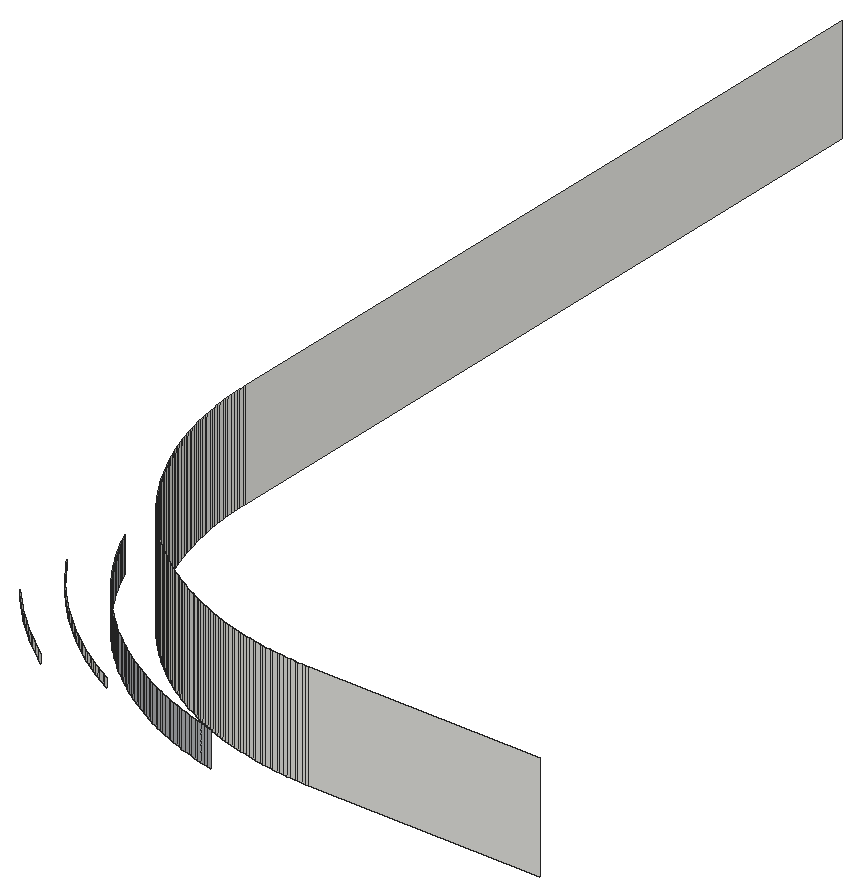
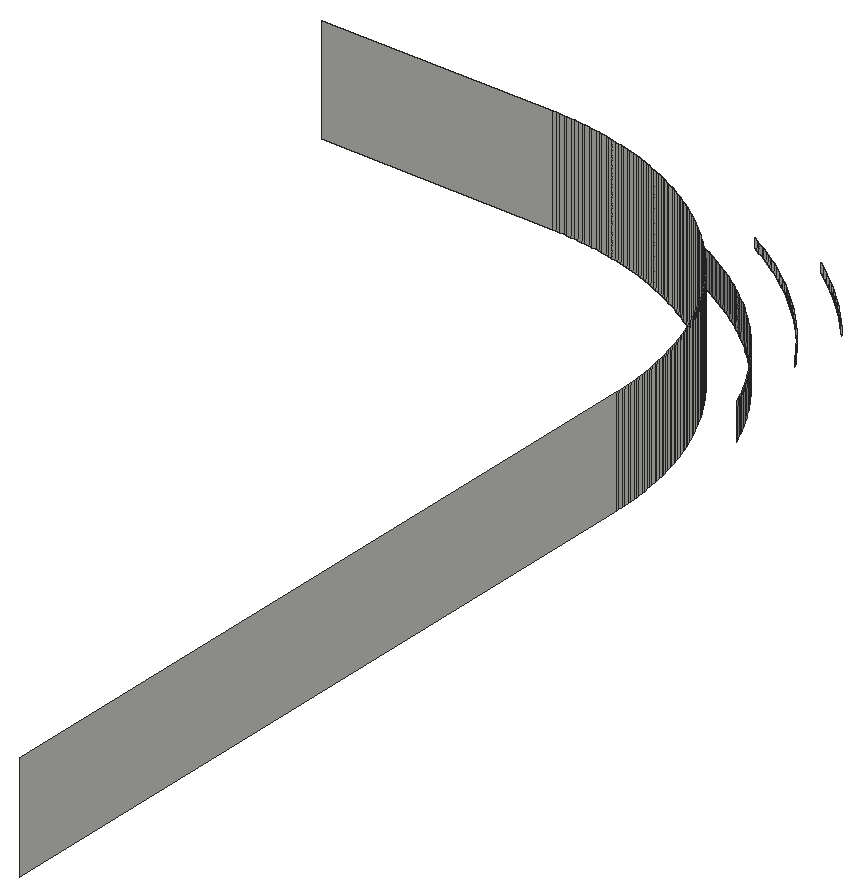
# SketchUp Ruby script. Lengths in inches.
U = 1.inch
M = Sketchup.active_model
def pt(a) = Geom::Point3d.new(a.map { |v| v * U })
def face(e, loops, mat)
  f = e.add_face(loops[0].map { |a| pt(a) })
  loops[1..].each { |l| e.add_face(l.map { |a| pt(a) }).erase! }
  f.material = f.back_material = mat if mat
  f
end
# faces: each face lists its corners as indices into pts; further lists are holes
def faces(e, pts, list, mat = nil) = list.each { |f| face(e, (f[0].is_a?(Array) ? f : [f]).map { |l| l.map { |i| pts[i] } }, mat) }
# xy, xz, yz: faces in a plane at the given z, y or x. An outline is a flat list of corners, or four numbers for a rectangle; further outlines are holes
def ring(l) = l.size == 4 ? [[l[0], l[1]], [l[2], l[1]], [l[2], l[3]], [l[0], l[3]]] : l.each_slice(2).to_a
def flat(e, list, mat, &to3) = list.each { |f| face(e, (f[0].is_a?(Array) ? f : [f]).map { |l| ring(l).map { |u, v| to3.(u, v) } }, mat) }
def xy(e, z, list, mat = nil) = flat(e, list, mat) { |x, y| [x, y, z] }
def xz(e, y, list, mat = nil) = flat(e, list, mat) { |x, z| [x, y, z] }
def yz(e, x, list, mat = nil) = flat(e, list, mat) { |y, z| [x, y, z] }
def lines(e, pts, list) = list.each { |a, b| e.add_line(pt(pts[a]), pt(pts[b])) }
# prism: a flat outline (further loops are holes) pulled along v
def prism(e, loops, v, mat = nil)
  f = face(e, loops, mat); d = Geom::Vector3d.new(v.map { |x| x * U })
  f.pushpull(f.normal.samedirection?(d) ? d.length : -d.length)
end
def box(e, o, s, mat = nil) = prism(e, [[o, [o[0] + s[0], o[1], o[2]], [o[0] + s[0], o[1] + s[1], o[2]], [o[0], o[1] + s[1], o[2]]]], [0, 0, s[2]], mat)
def at(x, y, z, deg = 0) = Geom::Transformation.translation(pt([x, y, z])) * Geom::Transformation.rotation(ORIGIN, Z_AXIS, deg.degrees)
def axes(o, x, y, z) = Geom::Transformation.new([*x, 0, *y, 0, *z, 0, *pt(o).to_a, 1])
def part(name) = M.definitions.add(name)
# library, detail: a bought-in or finely detailed component or shape, given as its bounding box
def library(name, o, s) = part(name).tap { |d| box(d.entities, o, s) }
def detail(e, o, s) = box(e.add_group.entities, o, s)
def put(e, d, t, mat = nil) = e.add_instance(d, t).tap { |i| i.material = mat if mat }
def group(e, t, mat = nil) = e.add_group.tap { |g| g.transformation = t; g.material = mat if mat }.entities
root = M.entities
M.materials.add("1427 AP 686 ARMOUR-N").color = [184, 186, 189]
xz(root,192,[[151.78,240,151.97,246],[151.97,240,165,246]])
xz(root,192.01,[[151.35,240,151.57,246]])
yz(root,134,[[209.78,240,209.97,246],[209.97,240,252,246]])
yz(root,134.01,[[209.35,240,209.57,246]])
p = [[147.21,190.58,240],[147.45,190.52,240],[147.45,190.52,242],[147.21,190.58,242],[147.68,190.47,240],[147.68,190.47,242],
  [146.75,190.7,240],[146.98,190.64,240],[146.98,190.64,242],[146.75,190.7,242],[146.51,190.77,240],[146.51,190.77,242],
  [146.05,190.91,240],[146.28,190.83,240],[146.28,190.83,242],[146.05,190.91,242],[145.82,190.98,240],[145.82,190.98,242],
  [145.59,191.05,240],[145.59,191.05,242],[145.13,191.22,240],[145.36,191.13,240],[145.36,191.13,242],[145.13,191.22,242],
  [144.91,191.3,240],[144.91,191.3,242],[144.68,191.39,240],[144.68,191.39,242],[144.46,191.48,240],[144.46,191.48,242],
  [144.23,191.57,240],[144.23,191.57,242],[144.01,191.66,240],[144.01,191.66,242],[143.79,191.76,240],[143.79,191.76,242],
  [143.57,191.86,240],[143.57,191.86,242],[143.35,191.97,240],[143.35,191.97,242],[143.14,192.07,240],[143.14,192.07,242],
  [150.48,192.0625,246],[150.7,192.05,246],[150.7,192.05,240],[150.48,192.0625,240],[150.91,192.03,246],[150.91,192.03,240],
  [151.13,192.02,246],[151.13,192.02,240],[151.35,192.01,246],[151.35,192.01,240],[151.57,192.01,246],[151.78,192,246],
  [151.78,192,240],[151.57,192.01,240],[142.92,192.18,240],[142.92,192.18,242],[149.61,192.16,246],[149.83,192.13,246],
  [149.83,192.13,240],[149.61,192.16,240],[150.05,192.11,246],[150.05,192.11,240],[150.26,192.08,246],[150.26,192.08,240],
  [142.71,192.29,240],[142.71,192.29,242],[148.97,192.26,246],[149.18,192.22,246],[149.18,192.22,240],[148.97,192.26,240],
  [149.4,192.1875,246],[149.4,192.1875,240],[142.49,192.4,240],[142.49,192.4,242],[148.33,192.38,246],[148.54,192.34,246],
  [148.54,192.34,240],[148.33,192.38,240],[148.76,192.29,246],[148.76,192.29,240],[142.28,192.52,240],[142.28,192.52,242],
  [147.9,192.47,246],[148.12,192.42,246],[148.12,192.42,240],[147.9,192.47,240],[142.07,192.64,240],[142.07,192.64,242],
  [147.48,192.58,246],[147.69,192.52,246],[147.69,192.52,240],[147.48,192.58,240],[141.86,192.76,240],[141.86,192.76,242],
  [147.0625,192.69,246],[147.27,192.63,246],[147.27,192.63,240],[147.0625,192.69,240],[146.85,192.75,246],[146.85,192.75,240],
  [141.65,192.88,240],[141.65,192.88,242],[146.4375,192.88,246],[146.64,192.81,246],[146.64,192.81,240],[146.4375,192.88,240],
  [141.45,193.01,240],[141.45,193.01,242],[146.03,193.02,246],[146.23,192.95,246],[146.23,192.95,240],[146.03,193.02,240],
  [141.24,193.14,240],[141.24,193.14,242],[145.82,193.09,246],[145.82,193.09,240],[141.04,193.27,240],[141.04,193.27,242],
  [145.62,193.17,246],[145.62,193.17,240],[145.21,193.33,246],[145.41,193.25,246],[145.41,193.25,240],[145.21,193.33,240],
  [140.84,193.4,240],[140.84,193.4,242],[145.01,193.41,246],[145.01,193.41,240],[140.64,193.54,240],[140.64,193.54,242],
  [144.8125,193.5,246],[144.8125,193.5,240],[140.44,193.68,240],[140.44,193.68,242],[144.61,193.59,246],[144.61,193.59,240],
  [144.41,193.68,246],[144.41,193.68,240],[140.24,193.82,240],[140.24,193.82,242],[144.22,193.77,246],[144.22,193.77,240],
  [140.05,193.96,240],[140.05,193.96,242],[144.02,193.86,246],[144.02,193.86,240],[143.83,193.96,246],[143.83,193.96,240],
  [139.86,194.11,240],[139.86,194.11,242],[143.63,194.0625,246],[143.63,194.0625,240],[139.67,194.26,240],[139.67,194.26,242],
  [143.44,194.16,246],[143.44,194.16,240],[143.25,194.27,246],[143.25,194.27,240],[139.48,194.41,240],[139.48,194.41,242],
  [143.0625,194.375,246],[143.0625,194.375,240],[139.29,194.56,240],[139.29,194.56,242],[142.875,194.48,246],[142.875,194.48,240],
  [142.6875,194.6,246],[142.6875,194.6,240],[139.1,194.71,240],[139.1,194.71,242],[142.5,194.71,246],[142.5,194.71,240],
  [138.92,194.87,240],[138.92,194.87,242],[142.32,194.83,246],[142.32,194.83,240],[142.14,194.94,246],[142.14,194.94,240],
  [138.74,195.03,240],[138.74,195.03,242],[141.95,195.0625,246],[141.95,195.0625,240],[138.56,195.19,240],[138.56,195.19,242],
  [141.77,195.1875,246],[141.77,195.1875,240],[138.38,195.35,240],[138.38,195.35,242],[141.6,195.3125,246],[141.6,195.3125,240],
  [141.42,195.4375,246],[141.42,195.4375,240],[138.2,195.52,240],[138.2,195.52,242],[141.24,195.57,246],[141.24,195.57,240],
  [138.03,195.6875,240],[138.03,195.6875,242],[141.07,195.7,246],[141.07,195.7,240],[137.86,195.86,240],[137.86,195.86,242],
  [140.9,195.83,246],[140.9,195.83,240],[140.73,195.97,246],[140.73,195.97,240],[137.6875,196.03,240],[137.6875,196.03,242],
  [137.52,196.2,240],[137.52,196.2,242],[140.56,196.1,246],[140.56,196.1,240],[140.39,196.24,246],[140.39,196.24,240],
  [137.35,196.38,240],[137.35,196.38,242],[140.23,196.38,246],[140.23,196.38,240],[137.19,196.56,240],[137.19,196.56,242],
  [140.0625,196.53,246],[140.0625,196.53,240],[139.9,196.67,246],[139.9,196.67,240],[137.03,196.74,240],[137.03,196.74,242],
  [136.87,196.92,240],[136.87,196.92,242],[139.74,196.82,246],[139.74,196.82,240],[139.58,196.97,246],[139.58,196.97,240],
  [136.71,197.1,240],[136.71,197.1,242],[139.43,197.12,246],[139.43,197.12,240],[136.56,197.29,240],[136.56,197.29,242],
  [139.27,197.27,246],[139.27,197.27,240],[136.41,197.48,240],[136.41,197.48,242],[139.12,197.43,246],[139.12,197.43,240],
  [138.97,197.58,246],[138.97,197.58,240],[136.26,197.67,240],[136.26,197.67,242],[138.82,197.74,246],[138.82,197.74,240],
  [136.11,197.86,240],[136.11,197.86,242],[138.67,197.9,246],[138.67,197.9,240],[135.96,198.05,240],[135.96,198.05,242],
  [138.53,198.0625,246],[138.53,198.0625,240],[135.82,198.24,240],[135.82,198.24,242],[138.38,198.23,246],[138.38,198.23,240],
  [135.68,198.44,240],[135.68,198.44,242],[138.24,198.39,246],[138.24,198.39,240],[135.54,198.64,240],[135.54,198.64,242],
  [138.1,198.56,246],[138.1,198.56,240],[135.4,198.84,240],[135.4,198.84,242],[137.97,198.73,246],[137.97,198.73,240],
  [137.83,198.9,246],[137.83,198.9,240],[135.27,199.04,240],[135.27,199.04,242],[137.7,199.07,246],[137.7,199.07,240],
  [135.14,199.24,240],[135.14,199.24,242],[137.57,199.24,246],[137.57,199.24,240],[135.01,199.45,240],[135.01,199.45,242],
  [137.4375,199.42,246],[137.4375,199.42,240],[134.88,199.65,240],[134.88,199.65,242],[137.3125,199.6,246],[137.3125,199.6,240],
  [137.1875,199.77,246],[137.1875,199.77,240],[134.76,199.86,240],[134.76,199.86,242],[137.0625,199.95,246],[137.0625,199.95,240],
  [134.64,200.07,240],[134.64,200.07,242],[136.94,200.14,246],[136.94,200.14,240],[134.52,200.28,240],[134.52,200.28,242],
  [136.83,200.32,246],[136.83,200.32,240],[134.4,200.49,240],[134.4,200.49,242],[136.71,200.5,246],[136.71,200.5,240],
  [134.29,200.71,240],[134.29,200.71,242],[136.6,200.6875,246],[136.6,200.6875,240],[134.18,200.92,240],[134.18,200.92,242],
  [136.48,200.875,246],[136.48,200.875,240],[134.07,201.14,240],[134.07,201.14,242],[136.375,201.0625,246],[136.375,201.0625,240],
  [133.97,201.35,240],[133.97,201.35,242],[136.27,201.25,246],[136.27,201.25,240],[136.16,201.44,246],[136.16,201.44,240],
  [133.86,201.57,240],[133.86,201.57,242],[136.0625,201.63,246],[136.0625,201.63,240],[133.76,201.79,240],[133.76,201.79,242],
  [135.96,201.83,246],[135.96,201.83,240],[135.86,202.02,246],[135.86,202.02,240],[135.77,202.22,246],[135.77,202.22,240],
  [135.68,202.41,246],[135.68,202.41,240],[135.59,202.61,246],[135.59,202.61,240],[135.5,202.8125,246],[135.5,202.8125,240],
  [135.41,203.01,246],[135.41,203.01,240],[135.33,203.21,246],[135.33,203.21,240],[135.25,203.41,246],[135.25,203.41,240],
  [135.17,203.62,246],[135.17,203.62,240],[135.09,203.82,246],[135.09,203.82,240],[135.02,204.03,246],[135.02,204.03,240],
  [134.95,204.23,246],[134.95,204.23,240],[134.88,204.4375,246],[134.88,204.4375,240],[134.81,204.64,246],[134.81,204.64,240],
  [134.75,204.85,246],[134.75,204.85,240],[134.69,205.0625,246],[134.69,205.0625,240],[134.63,205.27,246],[134.63,205.27,240],
  [134.58,205.48,246],[134.58,205.48,240],[134.52,205.69,246],[134.52,205.69,240],[134.47,205.9,246],[134.47,205.9,240],
  [134.42,206.12,246],[134.42,206.12,240],[134.38,206.33,246],[134.38,206.33,240],[134.34,206.54,246],[134.34,206.54,240],
  [134.29,206.76,246],[134.29,206.76,240],[134.26,206.97,246],[134.26,206.97,240],[134.22,207.18,246],[134.22,207.18,240],
  [134.1875,207.4,246],[134.1875,207.4,240],[134.16,207.61,246],[134.16,207.61,240],[134.13,207.83,246],[134.13,207.83,240],
  [134.11,208.05,246],[134.11,208.05,240],[134.08,208.26,246],[134.08,208.26,240],[134.0625,208.48,246],[134.0625,208.48,240],
  [134.05,208.7,246],[134.05,208.7,240],[134.03,208.91,246],[134.03,208.91,240],[134.02,209.13,246],[134.02,209.13,240],
  [134.01,209.35,246],[134.01,209.35,240],[134,209.78,246],[134.01,209.57,246],[134.01,209.57,240],[134,209.78,240],
  [138.13,190.41,242],[137.89,190.58,242],[137.89,190.58,242.5],[138.13,190.41,242.5],[141.54,190.64,242],[141.78,190.52,242],
  [141.78,190.52,242.5],[141.54,190.64,242.5],[137.66,190.76,242],[137.66,190.76,242.5],[141.31,190.77,242],[141.31,190.77,242.5],
  [137.43,190.93,242],[137.43,190.93,242.5],[141.08,190.9,242],[141.08,190.9,242.5],[137.2,191.11,242],[137.2,191.11,242.5],
  [140.85,191.04,242],[140.85,191.04,242.5],[140.62,191.17,242],[140.62,191.17,242.5],[136.97,191.29,242],[136.97,191.29,242.5],
  [140.39,191.3125,242],[140.39,191.3125,242.5],[136.75,191.47,242],[136.75,191.47,242.5],[140.17,191.45,242],[140.17,191.45,242.5],
  [136.52,191.66,242],[136.52,191.66,242.5],[139.94,191.6,242],[139.94,191.6,242.5],[139.72,191.74,242],[139.72,191.74,242.5],
  [136.3,191.84,242],[136.3,191.84,242.5],[139.5,191.89,242],[139.5,191.89,242.5],[136.08,192.04,242],[136.08,192.04,242.5],
  [139.28,192.05,242],[139.28,192.05,242.5],[135.87,192.23,242],[135.87,192.23,242.5],[139.07,192.2,242],[139.07,192.2,242.5],
  [135.66,192.43,242],[135.66,192.43,242.5],[138.85,192.36,242],[138.85,192.36,242.5],[135.44,192.625,242],[135.44,192.625,242.5],
  [138.64,192.52,242],[138.64,192.52,242.5],[138.43,192.68,242],[138.43,192.68,242.5],[135.24,192.83,242],[135.24,192.83,242.5],
  [138.22,192.85,242],[138.22,192.85,242.5],[135.03,193.03,242],[135.03,193.03,242.5],[138.02,193.01,242],[138.02,193.01,242.5],
  [134.83,193.24,242],[134.83,193.24,242.5],[137.8125,193.18,242],[137.8125,193.18,242.5],[134.625,193.44,242],[134.625,193.44,242.5],
  [137.61,193.36,242],[137.61,193.36,242.5],[134.43,193.66,242],[134.43,193.66,242.5],[137.41,193.53,242],[137.41,193.53,242.5],
  [137.21,193.71,242],[137.21,193.71,242.5],[134.23,193.87,242],[134.23,193.87,242.5],[137.02,193.89,242],[137.02,193.89,242.5],
  [134.04,194.08,242],[134.04,194.08,242.5],[136.82,194.07,242],[136.82,194.07,242.5],[133.84,194.3,242],[133.84,194.3,242.5],
  [136.63,194.26,242],[136.63,194.26,242.5],[136.44,194.44,242],[136.44,194.44,242.5],[136.26,194.63,242],[136.26,194.63,242.5],
  [136.07,194.82,242],[136.07,194.82,242.5],[135.89,195.02,242],[135.89,195.02,242.5],[135.71,195.21,242],[135.71,195.21,242.5],
  [135.53,195.41,242],[135.53,195.41,242.5],[135.36,195.61,242],[135.36,195.61,242.5],[135.18,195.8125,242],[135.18,195.8125,242.5],
  [135.01,196.02,242],[135.01,196.02,242.5],[134.85,196.22,242],[134.85,196.22,242.5],[134.68,196.43,242],[134.68,196.43,242.5],
  [134.52,196.64,242],[134.52,196.64,242.5],[134.36,196.85,242],[134.36,196.85,242.5],[134.2,197.07,242],[134.2,197.07,242.5],
  [134.05,197.28,242],[134.05,197.28,242.5],[133.89,197.5,242],[133.89,197.5,242.5],[133.74,197.72,242],[133.74,197.72,242.5]]
faces(root,p,[[0,1,2,3],[1,4,5,2],[6,7,8,9],[7,0,3,8],[10,6,9,11],[12,13,14,15],[13,10,11,14],[16,12,15,17],
  [18,16,17,19],[20,21,22,23],[21,18,19,22],[24,20,23,25],[26,24,25,27],[28,26,27,29],[30,28,29,31],[32,30,31,33],
  [34,32,33,35],[36,34,35,37],[38,36,37,39],[40,38,39,41],[56,40,41,57],[66,56,57,67],[74,66,67,75],[82,74,75,83],
  [88,82,83,89],[94,88,89,95],[102,94,95,103],[108,102,103,109],[114,108,109,115],[118,114,115,119],[126,118,119,127],[130,126,127,131],
  [134,130,131,135],[140,134,135,141],[144,140,141,145],[150,144,145,151],[154,150,151,155],[160,154,155,161],[164,160,161,165],[170,164,165,171],
  [174,170,171,175],[180,174,175,181],[184,180,181,185],[188,184,185,189],[194,188,189,195],[198,194,195,199],[202,198,199,203],[208,202,203,209],
  [210,208,209,211],[216,210,211,217],[220,216,217,221],[226,220,221,227],[228,226,227,229],[234,228,229,235],[238,234,235,239],[242,238,239,243],
  [248,242,243,249],[252,248,249,253],[256,252,253,257],[260,256,257,261],[264,260,261,265],[268,264,265,269],[272,268,269,273],[278,272,273,279],
  [282,278,279,283],[286,282,283,287],[290,286,287,291],[296,290,291,297],[300,296,297,301],[304,300,301,305],[308,304,305,309],[312,308,309,313],
  [316,312,313,317],[320,316,317,321],[324,320,321,325],[330,324,325,331],[334,330,331,335]],"1427 AP 686 ARMOUR-N")
faces(root,p,[[42,43,44,45],[43,46,47,44],[46,48,49,47],[48,50,51,49],[52,53,54,55],[58,59,60,61],[59,62,63,60],[62,64,65,63],
  [64,42,45,65],[68,69,70,71],[69,72,73,70],[72,58,61,73],[76,77,78,79],[77,80,81,78],[80,68,71,81],[84,85,86,87],
  [85,76,79,86],[90,91,92,93],[91,84,87,92],[96,97,98,99],[97,90,93,98],[100,96,99,101],[104,105,106,107],[105,100,101,106],
  [110,111,112,113],[111,104,107,112],[116,110,113,117],[120,116,117,121],[122,123,124,125],[123,120,121,124],[128,122,125,129],[132,128,129,133],
  [136,132,133,137],[138,136,137,139],[142,138,139,143],[146,142,143,147],[148,146,147,149],[152,148,149,153],[156,152,153,157],[158,156,157,159],
  [162,158,159,163],[166,162,163,167],[168,166,167,169],[172,168,169,173],[176,172,173,177],[178,176,177,179],[182,178,179,183],[186,182,183,187],
  [190,186,187,191],[192,190,191,193],[196,192,193,197],[200,196,197,201],[204,200,201,205],[206,204,205,207],[212,206,207,213],[214,212,213,215],
  [218,214,215,219],[222,218,219,223],[224,222,223,225],[230,224,225,231],[232,230,231,233],[236,232,233,237],[240,236,237,241],[244,240,241,245],
  [246,244,245,247],[250,246,247,251],[254,250,251,255],[258,254,255,259],[262,258,259,263],[266,262,263,267],[270,266,267,271],[274,270,271,275],
  [276,274,275,277],[280,276,277,281],[284,280,281,285],[288,284,285,289],[292,288,289,293],[294,292,293,295],[298,294,295,299],[302,298,299,303],
  [306,302,303,307],[310,306,307,311],[314,310,311,315],[318,314,315,319],[322,318,319,323],[326,322,323,327],[328,326,327,329],[332,328,329,333],
  [336,332,333,337],[338,336,337,339],[340,338,339,341],[342,340,341,343],[344,342,343,345],[346,344,345,347],[348,346,347,349],[350,348,349,351],
  [352,350,351,353],[354,352,353,355],[356,354,355,357],[358,356,357,359],[360,358,359,361],[362,360,361,363],[364,362,363,365],[366,364,365,367],
  [368,366,367,369],[370,368,369,371],[372,370,371,373],[374,372,373,375],[376,374,375,377],[378,376,377,379],[380,378,379,381],[382,380,381,383],
  [384,382,383,385],[386,384,385,387],[388,386,387,389],[390,388,389,391],[392,390,391,393],[394,392,393,395],[396,394,395,397],[398,396,397,399],
  [400,398,399,401],[402,400,401,403],[404,402,403,405],[406,404,405,407],[408,406,407,409],[410,411,412,413],[414,415,416,417],[418,419,420,421],
  [415,422,423,416],[424,418,421,425],[422,426,427,423],[428,424,425,429],[426,430,431,427],[432,428,429,433],[434,432,433,435],[430,436,437,431],
  [438,434,435,439],[436,440,441,437],[442,438,439,443],[440,444,445,441],[446,442,443,447],[448,446,447,449],[444,450,451,445],[452,448,449,453],
  [450,454,455,451],[456,452,453,457],[454,458,459,455],[460,456,457,461],[458,462,463,459],[464,460,461,465],[462,466,467,463],[468,464,465,469],
  [470,468,469,471],[466,472,473,467],[474,470,471,475],[472,476,477,473],[478,474,475,479],[476,480,481,477],[482,478,479,483],[480,484,485,481],
  [486,482,483,487],[484,488,489,485],[490,486,487,491],[492,490,491,493],[488,494,495,489],[496,492,493,497],[494,498,499,495],[500,496,497,501],
  [498,502,503,499],[504,500,501,505],[506,504,505,507],[508,506,507,509],[510,508,509,511],[512,510,511,513],[514,512,513,515],[516,514,515,517],
  [518,516,517,519],[520,518,519,521],[522,520,521,523],[524,522,523,525],[526,524,525,527],[528,526,527,529],[530,528,529,531],[532,530,531,533],
  [534,532,533,535],[536,534,535,537],[538,536,537,539]])
